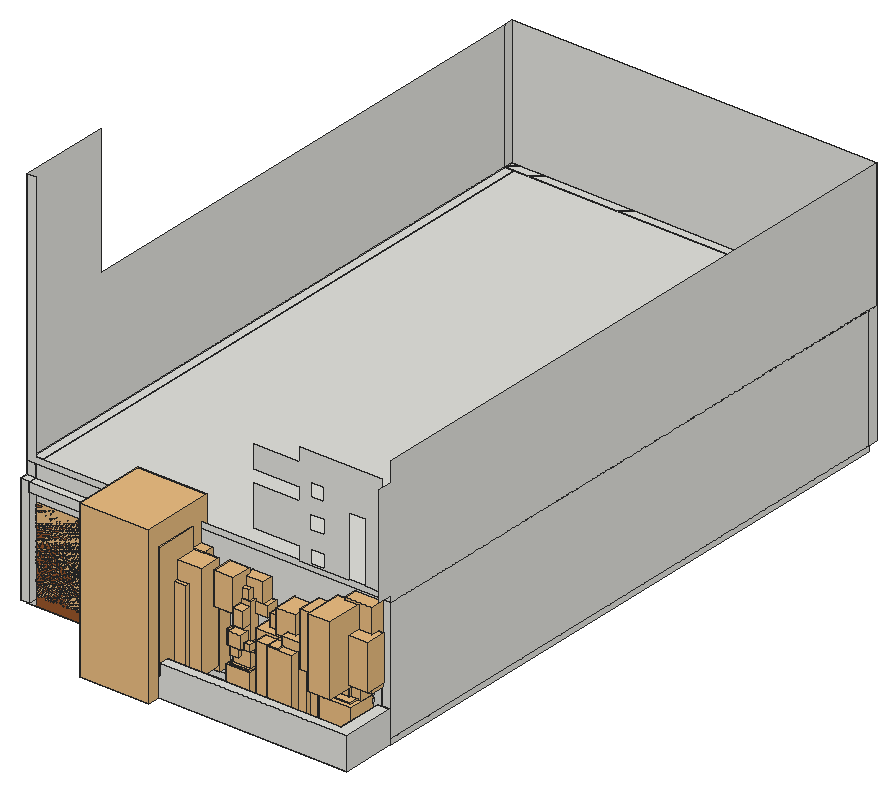
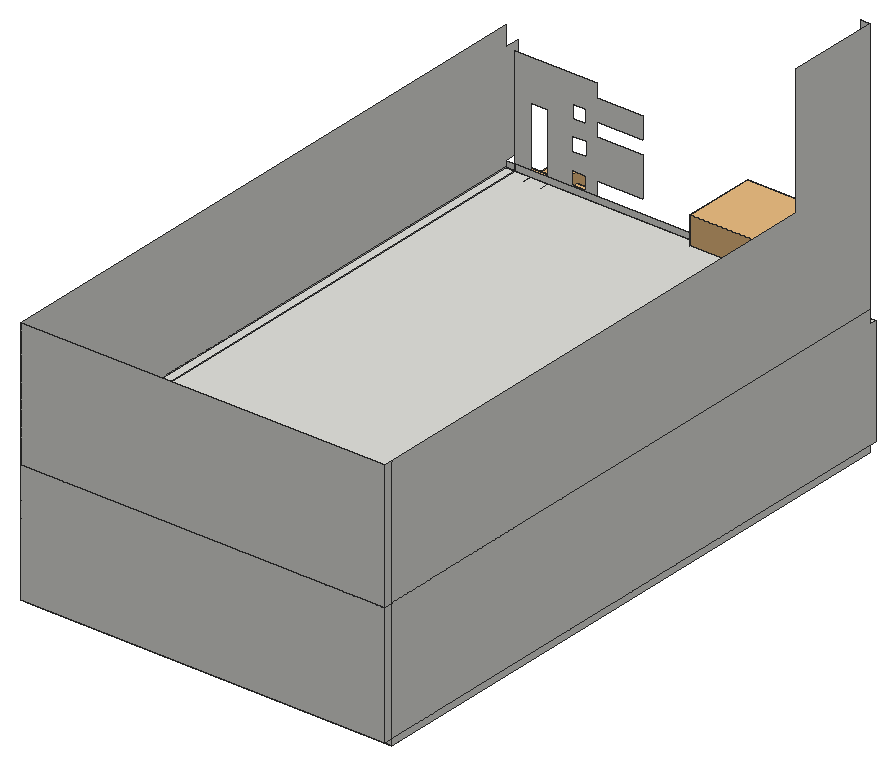
# SketchUp Ruby script. Lengths in inches.
U = 1.inch
M = Sketchup.active_model
def pt(a) = Geom::Point3d.new(a.map { |v| v * U })
def face(e, loops, mat)
  f = e.add_face(loops[0].map { |a| pt(a) })
  loops[1..].each { |l| e.add_face(l.map { |a| pt(a) }).erase! }
  f.material = f.back_material = mat if mat
  f
end
# faces: each face lists its corners as indices into pts; further lists are holes
def faces(e, pts, list, mat = nil) = list.each { |f| face(e, (f[0].is_a?(Array) ? f : [f]).map { |l| l.map { |i| pts[i] } }, mat) }
# xy, xz, yz: faces in a plane at the given z, y or x. An outline is a flat list of corners, or four numbers for a rectangle; further outlines are holes
def ring(l) = l.size == 4 ? [[l[0], l[1]], [l[2], l[1]], [l[2], l[3]], [l[0], l[3]]] : l.each_slice(2).to_a
def flat(e, list, mat, &to3) = list.each { |f| face(e, (f[0].is_a?(Array) ? f : [f]).map { |l| ring(l).map { |u, v| to3.(u, v) } }, mat) }
def xy(e, z, list, mat = nil) = flat(e, list, mat) { |x, y| [x, y, z] }
def xz(e, y, list, mat = nil) = flat(e, list, mat) { |x, z| [x, y, z] }
def yz(e, x, list, mat = nil) = flat(e, list, mat) { |y, z| [x, y, z] }
def lines(e, pts, list) = list.each { |a, b| e.add_line(pt(pts[a]), pt(pts[b])) }
# prism: a flat outline (further loops are holes) pulled along v
def prism(e, loops, v, mat = nil)
  f = face(e, loops, mat); d = Geom::Vector3d.new(v.map { |x| x * U })
  f.pushpull(f.normal.samedirection?(d) ? d.length : -d.length)
end
def box(e, o, s, mat = nil) = prism(e, [[o, [o[0] + s[0], o[1], o[2]], [o[0] + s[0], o[1] + s[1], o[2]], [o[0], o[1] + s[1], o[2]]]], [0, 0, s[2]], mat)
def at(x, y, z, deg = 0) = Geom::Transformation.translation(pt([x, y, z])) * Geom::Transformation.rotation(ORIGIN, Z_AXIS, deg.degrees)
def axes(o, x, y, z) = Geom::Transformation.new([*x, 0, *y, 0, *z, 0, *pt(o).to_a, 1])
def part(name) = M.definitions.add(name)
# library, detail: a bought-in or finely detailed component or shape, given as its bounding box
def library(name, o, s) = part(name).tap { |d| box(d.entities, o, s) }
def detail(e, o, s) = box(e.add_group.entities, o, s)
def put(e, d, t, mat = nil) = e.add_instance(d, t).tap { |i| i.material = mat if mat }
def group(e, t, mat = nil) = e.add_group.tap { |g| g.transformation = t; g.material = mat if mat }.entities
root = M.entities
M.materials.add("BANANA_BIG_STVOL_1").color = [93, 83, 53]
M.materials.add("POT_TEXTURE_1").color = [172, 172, 172]
M.materials.add("POT_TEXTURE_2").color = [160, 154, 144]
M.materials.add("[Translucent Glass Gray]").color = [128, 128, 128]
M.materials["[Translucent Glass Gray]"].alpha = 0.5
M.materials.add("[Wood Cherry Original]").color = [152, 86, 42]
M.materials.add("[Wood Floor]").color = [155, 105, 61]
M.materials.add("soil1").color = [68, 55, 47]
M.materials.add("wood_1").color = [140, 119, 94]
c1 = library("Plant",[-27.84,-31.84,-1.26],[68.28,70.82,154.38])
c2 = library("Group\#82",[-662.41,217.3,320.04],[397.32,658.3,1732.06])
c3 = library("Group\#84",[-299.2,181.55,262.58],[360.65,735.71,1258.34])
c4 = library("Group\#79",[-1038.76,656.55,345.34],[733.18,460.51,2065.7])
c5 = library("Group\#77",[-445.29,890.31,329.28],[284.3,304.08,2023.29])
c6 = library("Group\#80",[-733.48,439.625,202.64],[456.28,533.12,1536.78])
c7 = library("Group\#83",[-455.56,899.32,410.78],[341.21,610.33,1581.5])
c8 = library("Group\#76",[-516.34,626.77,-4.5625],[517.73,515.95,418.98])
c9 = library("Group\#81",[-249.24,914.85,310.18],[345.55,647.95,1307.93])
c10 = library("Group\#78",[-277.97,488.68,287.26],[362.84,405.94,1768.54])
c11 = library("Group\#75",[-468.76,669.89,380.1875],[424.36,427.47,41.99])
c12 = part("Potted broadleaf plant")
put(c12.entities,c2,at(1038.76,-181.55,4.5625))
put(c12.entities,c3,at(1038.76,-181.55,4.5625))
put(c12.entities,c4,at(1038.76,-181.55,4.5625))
put(c12.entities,c5,at(1038.76,-181.55,4.5625))
put(c12.entities,c6,at(1038.76,-181.55,4.5625))
put(c12.entities,c7,at(1038.76,-181.55,4.5625))
put(c12.entities,c8,at(1038.76,-181.55,4.5625),"POT_TEXTURE_1")
put(c12.entities,c9,at(1038.76,-181.55,4.5625))
put(c12.entities,c10,at(1038.76,-181.55,4.5625))
put(c12.entities,c11,at(1038.76,-181.55,4.5625),"soil1")
c13 = library("Group\#88",[-246.45,-349.05,558.47],[136.91,100.49,66.1])
c14 = library("Group\#91",[-264.68,-415.73,1484.11],[304.64,209.69,227.41])
c15 = library("Group\#98",[-357.04,-394.18,1447.05],[213.62,306.36,356.95])
c16 = library("Group\#86",[-447.02,-464.95,536.35],[343.73,346.24,39.39])
c17 = library("Group\#87",[-394.9,-448.99,911.74],[90.19,96.88,85.93])
c18 = library("Group\#97",[-424,-312.27,817.53],[158.81,108.06,136.45])
c19 = library("Group\#101",[-409.02,-515.05,915.53],[69.62,77.27,65.47])
c20 = library("Group\#105",[-548.25,-262.82,1459.54],[373.26,352.35,568])
c21 = library("Group\#112",[-492.14,-508.4,-4.15],[433.72,431.71,567.03])
c22 = library("Group\#108",[-293.78,-482.77,597.9],[158.75,112.78,159.87])
c23 = library("Group\#92",[-545.09,-386.51,922.3125],[300.25,219.65,227.33])
c24 = library("Group\#110",[-292.81,-667.38,1418.14],[215.17,356.07,188.87])
c25 = library("Group\#94",[-292.14,-288.9,1281.79],[169.55,204.34,203.36])
c26 = library("Group\#99",[-568.91,-444.37,1285.4],[307.6,179.39,277.93])
c27 = library("Group\#96",[-341.93,-403.49,744.8125],[64.83,96.32,132.15])
c28 = library("Group\#85",[-258.04,-282.68,604.05],[115.53,137.01,52.63])
c29 = library("Group\#93",[-304.79,-269.16,622.65],[82.06,111.89,102.57])
c30 = library("Group\#100",[-388.93,-514.39,838.93],[89.79,77.73,82.08])
c31 = library("Group\#102",[-295.03,-516.52,742.34],[68.71,141.75,78.67])
c32 = library("Group\#109",[-422.77,-235.4,843.61],[178.54,197.77,233.54])
c33 = library("Group\#103",[-498.98,-524.4,908.45],[120.83,107.95,112.98])
c34 = library("Group\#106",[-321.08,-139.66,1308.49],[285.55,393.29,221.53])
c35 = library("Group\#104",[-278.4,-571.99,1530.91],[311.57,345.77,423.62])
c36 = library("Group\#107",[-387.74,-136.11,1470.07],[230,321.58,230.27])
c37 = library("Group\#95",[-244.55,-305.59,1009.46],[103.13,76.81,77.34])
c38 = library("Group\#111",[-385.21,-446.52,494.02],[160.93,321.12,1142.36])
c39 = library("Group\#89",[-249.18,-250.59,980.93],[152.21,116.16,134.05])
c40 = library("Group\#90",[-438.92,-265.61,702.3],[171.52,146.16,133.5])
c41 = part("Potted broadleaf tree")
p = [[568.91,667.38,4.15],[569.91,667.38,4.15],[569.91,668.38,4.15]]
lines(c41.entities,p,[[0,1],[1,2],[2,0]])
put(c41.entities,c13,at(568.91,667.38,4.15))
put(c41.entities,c14,at(568.91,667.38,4.15))
put(c41.entities,c15,at(568.91,667.38,4.15))
put(c41.entities,c16,at(568.91,667.38,4.15),"soil1")
put(c41.entities,c17,at(568.91,667.38,4.15))
put(c41.entities,c18,at(568.91,667.38,4.15))
put(c41.entities,c19,at(568.91,667.38,4.15))
put(c41.entities,c20,at(568.91,667.38,4.15))
put(c41.entities,c21,at(568.91,667.38,4.15),"POT_TEXTURE_2")
put(c41.entities,c22,at(568.91,667.38,4.15))
put(c41.entities,c23,at(568.91,667.38,4.15))
put(c41.entities,c24,at(568.91,667.38,4.15))
put(c41.entities,c25,at(568.91,667.38,4.15))
put(c41.entities,c26,at(568.91,667.38,4.15))
put(c41.entities,c27,at(568.91,667.38,4.15))
put(c41.entities,c28,at(568.91,667.38,4.15))
put(c41.entities,c29,at(568.91,667.38,4.15))
put(c41.entities,c30,at(568.91,667.38,4.15))
put(c41.entities,c31,at(568.91,667.38,4.15))
put(c41.entities,c32,at(568.91,667.38,4.15))
put(c41.entities,c33,at(568.91,667.38,4.15))
put(c41.entities,c34,at(568.91,667.38,4.15))
put(c41.entities,c35,at(568.91,667.38,4.15))
put(c41.entities,c36,at(568.91,667.38,4.15))
put(c41.entities,c37,at(568.91,667.38,4.15))
put(c41.entities,c38,at(568.91,667.38,4.15),"wood_1")
put(c41.entities,c39,at(568.91,667.38,4.15))
put(c41.entities,c40,at(568.91,667.38,4.15))
c42 = library("Group\#120",[-640.625,-1318.37,287.11],[396.64,314.81,689.96])
c43 = library("Group\#115",[-513.94,-1201.2,195.17],[480.66,557.42,1160.08])
c44 = library("Group\#117",[-208.03,-1336.63,286.21],[381.72,484.79,1145.39])
c45 = library("Group\#123",[-619.83,-1636.3,288.9],[316.15,456.61,1171.28])
c46 = library("Group\#124",[-738.91,-1210.08,301],[426.4,388.88,1000.79])
c47 = library("Group\#126",[-208.33,-1511.76,297.04],[508.2,421.96,1258.76])
c48 = library("Group\#116",[-545.36,-1775.03,287.125],[412.21,432,920.68])
c49 = library("Group\#121",[-750.24,-1478.51,301.56],[423.84,451.05,998.69])
c50 = library("Group\#119",[-245.33,-1174.2,301.22],[356.02,306.31,608.34])
c51 = library("Group\#114",[-487.23,-1483.58,-4.71],[450.86,446.99,418.38])
c52 = library("Group\#128",[-445.7,-1606.55,154.18],[255.44,283.57,849.28])
c53 = library("Group\#129",[-390.1,-1177.12,195.59],[220.93,265.44,790.12])
c54 = library("Group\#131",[-480.32,-1333.42,295.8],[424.49,356.06,1482.77])
c55 = library("Group\#132",[-378.01,-1245.98,305.66],[422.15,474.55,1267.42])
c56 = library("Group\#118",[-163.65,-1622.09,292.29],[406.18,374.8,780.12])
c57 = library("Group\#127",[-384.8,-1640.99,300.61],[422.68,348.03,1297.96])
c58 = library("Group\#113",[-429.18,-1441.17,362.05],[345.84,348.28,45.35])
c59 = library("Group\#130",[-208.0625,-1498.77,286.27],[547.26,435.76,1075.6])
c60 = library("Group\#125",[-172.82,-1329.68,294.68],[502.85,397.72,955.79])
c61 = library("Group\#122",[-426.76,-1753.59,287.48],[479.67,412.35,1049.19])
c62 = part("Potted palm")
put(c62.entities,c42,at(750.24,1775.03,4.71))
put(c62.entities,c43,at(750.24,1775.03,4.71))
put(c62.entities,c44,at(750.24,1775.03,4.71))
put(c62.entities,c45,at(750.24,1775.03,4.71))
put(c62.entities,c46,at(750.24,1775.03,4.71))
put(c62.entities,c47,at(750.24,1775.03,4.71))
put(c62.entities,c48,at(750.24,1775.03,4.71))
put(c62.entities,c49,at(750.24,1775.03,4.71))
put(c62.entities,c50,at(750.24,1775.03,4.71))
put(c62.entities,c51,at(750.24,1775.03,4.71),"POT_TEXTURE_1")
put(c62.entities,c52,at(750.24,1775.03,4.71))
put(c62.entities,c53,at(750.24,1775.03,4.71))
put(c62.entities,c54,at(750.24,1775.03,4.71))
put(c62.entities,c55,at(750.24,1775.03,4.71))
put(c62.entities,c56,at(750.24,1775.03,4.71))
put(c62.entities,c57,at(750.24,1775.03,4.71))
put(c62.entities,c58,at(750.24,1775.03,4.71),"soil1")
put(c62.entities,c59,at(750.24,1775.03,4.71))
put(c62.entities,c60,at(750.24,1775.03,4.71))
put(c62.entities,c61,at(750.24,1775.03,4.71))
c63 = library("Group\#133",[-480.3,-2300.47,677.45],[398.14,398.43,28.25])
c64 = library("Group\#134",[-336.38,-2175.79,614.41],[133.99,147.1,560.64])
c65 = library("Group\#135",[-311.45,-2362.85,663.67],[597.01,322.07,1007.38])
c66 = library("Group\#136",[-330.26,-2159.14,612.04],[116.66,119.22,673.97])
c67 = library("Group\#137",[-667.53,-2111.4375,1071.74],[420.02,555.28,968.03])
c68 = library("Group\#138",[-328.97,-2115.58,1156.29],[117.86,119.42,695.38])
c69 = library("Group\#139",[-943.22,-2312.1875,967.59],[670.63,402.45,1245.73])
c70 = library("Group\#141",[-343.93,-2076.42,1024.91],[285.05,475.82,708.21])
c71 = library("Group\#140",[-568.09,-2386.9,-3.76],[573.62,569.18,700.28])
c72 = library("Group\#142",[-550.09,-2664.39,1031.96],[371.42,533.86,798])
c73 = library("Group\#143",[-308.37,-2556.11,869.35],[483.58,483.6,1385.8])
c74 = part("Potted broadleaf plant \#1")
put(c74.entities,c63,at(943.22,2664.39,3.76),"soil1")
put(c74.entities,c64,at(943.22,2664.39,3.76),"BANANA_BIG_STVOL_1")
put(c74.entities,c65,at(943.22,2664.39,3.76))
put(c74.entities,c66,at(943.22,2664.39,3.76),"BANANA_BIG_STVOL_1")
put(c74.entities,c67,at(943.22,2664.39,3.76))
put(c74.entities,c68,at(943.22,2664.39,3.76))
put(c74.entities,c69,at(943.22,2664.39,3.76))
put(c74.entities,c70,at(943.22,2664.39,3.76))
put(c74.entities,c71,at(943.22,2664.39,3.76),"POT_TEXTURE_2")
put(c74.entities,c72,at(943.22,2664.39,3.76))
put(c74.entities,c73,at(943.22,2664.39,3.76))
c75 = part("plants")
put(c75.entities,c12,at(-1038.76,181.55,-4.5625))
put(c75.entities,c41,at(-568.91,-667.38,-4.15))
put(c75.entities,c62,at(-750.24,-1775.03,-4.71))
put(c75.entities,c74,at(-943.22,-2664.39,-3.76))
c76 = library("Modern Gate 1",[0,0,0],[118.11,1.97,78.74])
c77 = part("window full")
xy(c77.entities,0,[[0,0,14.17,66.54]])
xy(c77.entities,2.26,[[12.2,2.26,14.17,64.28]],"[Wood Floor]")
xy(c77.entities,2.36,[[0,2.36,1.97,64.17]],"[Wood Floor]")
xy(c77.entities,3.74,[[11.42,3.74,12.2,32.875],[11.42,33.66,12.2,62.79]],"[Wood Floor]")
xy(c77.entities,3.9375,[[1.97,3.9375,2.76,32.77],[1.97,33.76,2.76,62.6]],"[Wood Floor]")
xy(c77.entities,4.18,[[2.76,4.18,7.09,32.09],[7.09,4.18,11.42,32.09],[2.76,34.45,7.09,62.35],[7.09,34.45,11.42,62.35]],"[Wood Floor]")
xy(c77.entities,69.83,[[2.76,4.18,7.09,32.09],[7.09,32.09,11.42,34.45],[2.76,34.45,7.09,62.35]])
xy(c77.entities,69.83,[[7.09,4.18,11.42,32.09],[7.09,34.45,11.42,62.35]],"[Wood Floor]")
xy(c77.entities,70.08,[[1.97,3.9375,2.76,32.77],[1.97,33.76,2.76,62.6]])
xy(c77.entities,70.27,[[11.42,32.875,12.2,33.66]])
xy(c77.entities,70.27,[[11.42,3.74,12.2,32.875],[11.42,33.66,12.2,62.79]],"[Wood Floor]")
xy(c77.entities,71.65,[[0,2.36,1.97,64.17]])
xy(c77.entities,71.76,[[12.2,2.26,14.17,64.28]],"[Wood Floor]")
xy(c77.entities,74.02,[[0,0,14.17,66.54]],"[Wood Floor]")
xz(c77.entities,0,[[0,0,14.17,74.02]],"[Wood Floor]")
xz(c77.entities,2.26,[[12.2,2.26,14.17,71.76]],"[Wood Floor]")
xz(c77.entities,2.36,[[0,2.36,1.97,71.65]],"[Wood Floor]")
xz(c77.entities,3.74,[[11.42,3.74,12.2,70.27]],"[Wood Floor]")
xz(c77.entities,3.9375,[[1.97,3.9375,2.76,70.08]],"[Wood Floor]")
xz(c77.entities,4.18,[[2.76,4.18,7.09,69.83],[7.09,4.18,11.42,69.83]],"[Wood Floor]")
xz(c77.entities,32.09,[[2.76,4.18,11.42,69.83]],"[Wood Floor]")
xz(c77.entities,32.77,[[1.97,3.9375,2.76,70.08]],"[Wood Floor]")
xz(c77.entities,32.875,[[11.42,3.74,12.2,70.27]],"[Wood Floor]")
xz(c77.entities,33.66,[[11.42,3.74,12.2,47.88],[11.42,47.88,12.2,70.27]],"[Wood Floor]")
xz(c77.entities,33.76,[[1.97,3.9375,2.76,70.08]],"[Wood Floor]")
xz(c77.entities,34.45,[[2.76,4.18,11.42,69.83]],"[Wood Floor]")
xz(c77.entities,62.35,[[2.76,4.18,7.09,69.83],[7.09,4.18,11.42,69.83]],"[Wood Floor]")
xz(c77.entities,62.6,[[1.97,3.9375,2.76,70.08]],"[Wood Floor]")
xz(c77.entities,62.79,[[11.42,3.74,12.2,70.27]],"[Wood Floor]")
xz(c77.entities,64.17,[[0,2.36,1.97,71.65]],"[Wood Floor]")
xz(c77.entities,64.28,[[12.2,2.26,14.17,71.76]],"[Wood Floor]")
xz(c77.entities,66.54,[[0,0,14.17,74.02]],"[Wood Floor]")
yz(c77.entities,0,[[[0,0,66.54,74.02],[2.36,2.36,64.17,71.65]]],"[Wood Floor]")
yz(c77.entities,1.97,[[[2.36,2.36,64.17,71.65],[33.76,3.9375,62.6,70.08],[3.9375,3.9375,32.77,70.08]]],"[Wood Floor]")
yz(c77.entities,2.76,[[32.77,3.9375,33.76,4.18],[32.77,4.18,33.76,69.83],[32.77,69.83,33.76,70.08]])
yz(c77.entities,2.76,[[[3.9375,3.9375,32.77,70.08],[4.18,4.18,32.09,69.83]],[[33.76,3.9375,62.6,70.08],[34.45,4.18,62.35,69.83]]],"[Wood Floor]")
yz(c77.entities,7.09,[[4.18,4.18,62.35,69.83]],"[Translucent Glass Gray]")
yz(c77.entities,11.42,[[32.875,69.83,33.66,70.27]])
yz(c77.entities,11.42,[[[3.74,3.74,32.875,70.27],[4.18,4.18,32.09,69.83]],[[33.66,3.74,62.79,70.27],[34.45,4.18,62.35,69.83]]],"[Wood Floor]")
yz(c77.entities,12.2,[[[2.26,2.26,64.28,71.76],[3.74,3.74,32.875,70.27],[33.66,3.74,62.79,70.27]]],"[Wood Floor]")
yz(c77.entities,14.17,[[[0,0,66.54,74.02],[2.26,2.26,64.28,71.76]]],"[Wood Floor]")
p = [[11.42,32.875,70.27],[11.42,32.875,70.28]]
lines(c77.entities,p,[[0,1]])
box(root,[316.53,51.4375,10.8],[27.06,2,3.38])
box(root,[316.53,51.4375,16.11],[27.06,2,3.38])
box(root,[316.53,51.4375,26.68],[27.06,2,3.37])
box(root,[316.53,51.4375,32.36],[27.06,2,3.38])
box(root,[316.53,51.4375,41.99],[27.06,2,3.37])
box(root,[316.53,51.4375,48.49],[27.06,2,3.37])
box(root,[316.53,51.4375,56.18],[27.06,2,3.37])
box(root,[316.53,51.4375,60.95],[27.06,2,3.38])
box(root,[316.53,51.4375,70.58],[27.06,2,3.37])
box(root,[316.53,51.4375,76.33],[27.06,2,3.37])
box(root,[316.53,51.4375,85.13],[27.06,2,3.38])
box(root,[316.53,51.4375,90.07],[27.06,2,3.38])
box(root,[316.53,51.4375,97.51],[27.06,2,3.37])
box(root,[316.53,51.4375,102.2],[27.06,2,3.37])
xy(root,-6,[[113.65,0,113.65,53.4375,126.09,53.4375,126.09,8.63,346.9,8.63,346.9,53.4375,359.34,53.4375,359.34,0],[126.09,8.63,346.9,53.4375],[0,53.4375,360,644.4375]])
xy(root,0,[[90,45.1875,101.25,53.4375],[0,45.6875,9,53.4375],[0,53.4375,9,644.4375]])
xy(root,25.5,[[113.65,0,359.34,0,359.34,53.4375,346.9,53.4375,346.9,8.63,126.09,8.63,126.09,53.4375,113.65,53.4375]])
xy(root,45.18,[[258.83,44,301.83,178.9375]])
xy(root,83.43,[[258.83,44,301.83,178.9375]])
xy(root,98.57,[[9,45.1875,9,453.625,101.25,453.625,101.25,53.4375,90,53.4375,90,45.1875],[90,45.1875,101.25,53.4375]])
xy(root,107.38,[[9,45.1875,101.25,453.625],[0,45.6875,9,53.4375]])
xy(root,120,[[0,53.4375,9,53.875],[351,53.4375,351,53.875,9,53.875,9,644.4375,0,644.4375,0,653.4375,360,653.4375,360,53.4375],[9,53.4375,318.32,53.875],[335.64,53.4375,351,53.875],[0,53.875,9,62.4375],
  [0,62.4375,9,644.4375]])
xz(root,0,[[113.65,-6,359.34,25.5]])
xz(root,8.63,[[126.09,-6,346.9,25.5]])
xz(root,44,[[[258.83,45.18,301.83,83.43],[261.66,48.51,299,80.6]]])
xz(root,45.1875,[[90,0,101.25,98.57],[9,98.57,101.25,107.38]])
xz(root,45.6875,[[0,0,9,107.38]])
xz(root,53.4375,[[0,-6,9,0],[90,-6,101.25,0],[101.25,-6,113.65,0],[113.65,-6,126.09,0],[126.09,-6,346.9,0],
  [346.9,-6,351,0],[351,-6,359.34,0],[359.34,-6,360,0],[90,0,101.25,98.57],[113.65,0,126.09,25.5],
  [346.9,0,351,25.5],[351,0,359.34,25.5],[0,107.38,9,120],[[351,120,360,120,360,126.125,351,126.125,351,226.37,270.3125,226.37,270.3125,213.25,224.5625,213.25,224.5625,191.52,270.3125,191.52,270.3125,178.4,224.5625,178.4,224.5625,139.25,270.3125,139.25,270.3125,126.125,318.32,126.125,318.32,185.5,335.64,185.5,335.64,126.125,351,126.125],[280.4375,156.97,294.5,171.03],[281.07,127.16,294.45,140.53],[281.15,186.3,294.21,199.36]]])
xz(root,53.4375,[[9,-6,90,84]],"[Wood Cherry Original]")
xz(root,53.875,[[0,120,351,120,351,126.125,9.02,126.125,9.02,373.61,0,373.61]])
xz(root,178.9375,[[[226.49,13.34,334.16,115.77],[258.83,45.18,301.83,83.43]],[[258.83,45.18,301.83,83.43],[265.1,51.95,295.56,77.16]],[265.1,51.95,295.56,77.16]])
xz(root,453.625,[[9,98.57,101.25,107.38]])
xz(root,644.4375,[[0,-6,360,0],[0,0,9,120]])
xz(root,653.4375,[[0,120,360,246]])
yz(root,0,[[53.4375,-6,644.4375,0],[45.6875,0,45.6875,107.38,53.4375,107.38,53.4375,120,644.4375,120,644.4375,0],[53.875,120,53.875,373.61,144.86,373.61,144.86,246,644.4375,246,644.4375,120],[644.4375,120,653.4375,246]])
yz(root,9,[[45.6875,0,644.4375,0,644.4375,120,53.4375,120,53.4375,107.38,453.625,107.38,453.625,98.57,45.6875,98.57],[45.1875,98.57,45.6875,107.38],[45.6875,98.57,453.625,107.38]])
yz(root,90,[[45.1875,0,53.4375,98.57]])
yz(root,101.25,[[45.1875,0,53.4375,98.57],[45.1875,98.57,453.625,107.38]])
yz(root,113.65,[[0,-6,53.4375,25.5]])
yz(root,126.09,[[8.63,-6,53.4375,25.5]])
yz(root,258.83,[[44,45.18,178.9375,83.43]])
yz(root,301.83,[[44,45.18,178.9375,83.43]])
yz(root,346.9,[[8.63,-6,53.4375,25.5]])
yz(root,351,[[53.4375,120,53.875,126.125]])
yz(root,359.34,[[0,-6,53.4375,25.5]])
yz(root,360,[[53.4375,-6,644.4375,0],[53.4375,120,653.4375,120,653.4375,246,53.875,246,53.4375,226.37,38.75,226.37,38.75,126.125,53.4375,126.125]])
p = [[318.32,53.875,120],[318.32,62.4375,120],[318.32,62.4375,87.31],[335.64,62.4375,87.31],[335.64,62.4375,120],[335.64,53.875,120],
  [318.32,53.4375,87.31],[318.32,53.875,87.31],[335.64,53.4375,87.31],[335.64,53.875,87.31],[351,53.4375,25.5],[351,53.4375,120]]
lines(root,p,[[0,1],[2,1],[3,2],[4,3],[4,5],[6,7],[8,9],[7,2],[9,3],[10,11]])
put(root,c1,at(131.89,21.46,-6))
put(root,c75,axes([210.9,57.38,-5.74],[0,0.05524,0],[-0.05524,0,0],[0,0,0.05524]))
g1 = group(root,at(0,644.4375,0))
box(g1,[0,0,0],[360,9,120])
g2 = group(root,at(351,53.4375,0))
box(g2,[0,0,0],[9,591,120])
g3 = group(root,at(9,53.4375,0))
xz(g3,0,[[81,0,342,0,342,120,0,120,0,84,81,84]])
put(root,c76,axes([9,53.4375,2.88],[0.68376,0,0],[0,0.67,0],[0,0,1.0586]),"[Wood Cherry Original]")
put(root,c77,axes([262.4,58.17,48.51],[0,-1,0],[0.55,0,0],[0,0,0.43357]))
